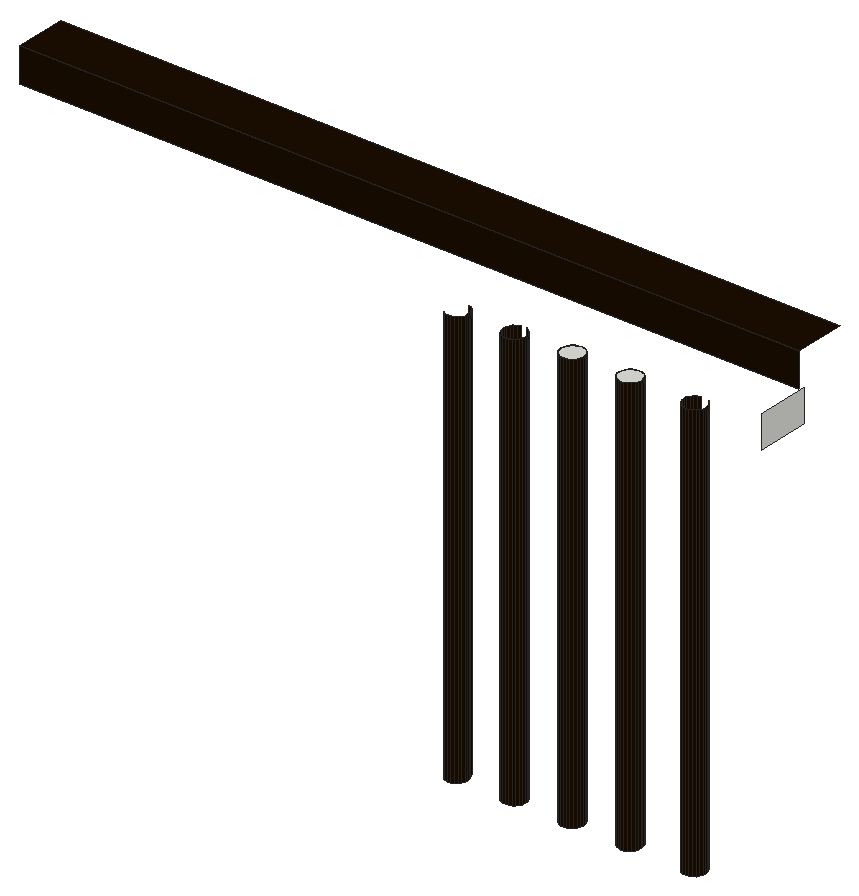
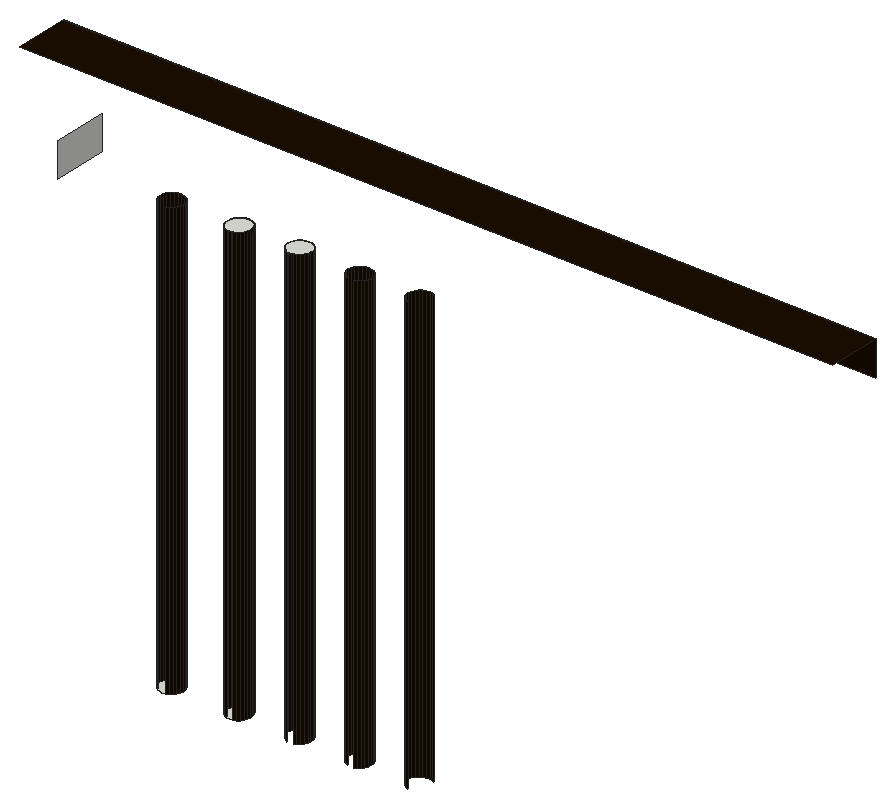
# SketchUp Ruby script. Lengths in inches.
U = 1.inch
M = Sketchup.active_model
def pt(a) = Geom::Point3d.new(a.map { |v| v * U })
def face(e, loops, mat)
  f = e.add_face(loops[0].map { |a| pt(a) })
  loops[1..].each { |l| e.add_face(l.map { |a| pt(a) }).erase! }
  f.material = f.back_material = mat if mat
  f
end
# faces: each face lists its corners as indices into pts; further lists are holes
def faces(e, pts, list, mat = nil) = list.each { |f| face(e, (f[0].is_a?(Array) ? f : [f]).map { |l| l.map { |i| pts[i] } }, mat) }
# xy, xz, yz: faces in a plane at the given z, y or x. An outline is a flat list of corners, or four numbers for a rectangle; further outlines are holes
def ring(l) = l.size == 4 ? [[l[0], l[1]], [l[2], l[1]], [l[2], l[3]], [l[0], l[3]]] : l.each_slice(2).to_a
def flat(e, list, mat, &to3) = list.each { |f| face(e, (f[0].is_a?(Array) ? f : [f]).map { |l| ring(l).map { |u, v| to3.(u, v) } }, mat) }
def xy(e, z, list, mat = nil) = flat(e, list, mat) { |x, y| [x, y, z] }
def xz(e, y, list, mat = nil) = flat(e, list, mat) { |x, z| [x, y, z] }
def yz(e, x, list, mat = nil) = flat(e, list, mat) { |y, z| [x, y, z] }
def lines(e, pts, list) = list.each { |a, b| e.add_line(pt(pts[a]), pt(pts[b])) }
# prism: a flat outline (further loops are holes) pulled along v
def prism(e, loops, v, mat = nil)
  f = face(e, loops, mat); d = Geom::Vector3d.new(v.map { |x| x * U })
  f.pushpull(f.normal.samedirection?(d) ? d.length : -d.length)
end
def box(e, o, s, mat = nil) = prism(e, [[o, [o[0] + s[0], o[1], o[2]], [o[0] + s[0], o[1] + s[1], o[2]], [o[0], o[1] + s[1], o[2]]]], [0, 0, s[2]], mat)
def at(x, y, z, deg = 0) = Geom::Transformation.translation(pt([x, y, z])) * Geom::Transformation.rotation(ORIGIN, Z_AXIS, deg.degrees)
def axes(o, x, y, z) = Geom::Transformation.new([*x, 0, *y, 0, *z, 0, *pt(o).to_a, 1])
def part(name) = M.definitions.add(name)
# library, detail: a bought-in or finely detailed component or shape, given as its bounding box
def library(name, o, s) = part(name).tap { |d| box(d.entities, o, s) }
def detail(e, o, s) = box(e.add_group.entities, o, s)
def put(e, d, t, mat = nil) = e.add_instance(d, t).tap { |i| i.material = mat if mat }
def group(e, t, mat = nil) = e.add_group.tap { |g| g.transformation = t; g.material = mat if mat }.entities
root = M.entities
M.materials.add("[Metal Seamed]1").color = [28, 14, 0]
xy(root,618.25,[[344.39,68.79,344.05,68.83,343.73,68.97,343.46,69.17,343.25,69.45,343.12,69.76,343.07,70.1,343.12,70.44,343.25,70.76,343.46,71.03,343.73,71.24,344.05,71.37,344.39,71.41,344.73,71.37,345.04,71.24,345.31,71.03,345.52,70.76,345.65,70.44,345.7,70.1,345.65,69.76,345.52,69.45,345.31,69.17,345.04,68.97,344.73,68.83],[351.89,68.79,351.55,68.83,351.23,68.97,350.96,69.17,350.75,69.45,350.62,69.76,350.58,70.1,350.62,70.44,350.75,70.76,350.96,71.03,351.23,71.24,351.55,71.37,351.89,71.41,352.23,71.37,352.55,71.24,352.82,71.03,353.03,70.76,353.16,70.44,353.2,70.1,353.16,69.76,353.03,69.45,352.82,69.17,352.55,68.97,352.23,68.83]])
xy(root,666.8125,[[344.39,68.79,344.73,68.83,345.04,68.97,345.31,69.17,345.52,69.45,345.65,69.76,345.7,70.1,345.65,70.44,345.52,70.76,345.31,71.03,345.04,71.24,344.73,71.37,344.39,71.41,344.05,71.37,343.73,71.24,343.46,71.03,343.25,70.76,343.12,70.44,343.07,70.1,343.12,69.76,343.25,69.45,343.46,69.17,343.73,68.97,344.05,68.83]])
xy(root,666.9375,[[337.7,68.79,338.04,68.83,338.36,68.97,338.63,69.17,338.84,69.45,338.97,69.76,339.01,70.1,338.97,70.44,338.84,70.76,338.63,71.03,338.36,71.24,338.04,71.37,337.7,71.41,337.36,71.37,337.04,71.24,336.77,71.03,336.5625,70.76,336.43,70.44,336.39,70.1,336.43,69.76,336.5625,69.45,336.77,69.17,337.04,68.97,337.36,68.83]])
xy(root,678.3125,[[275.92,67.28,366.15,73.28]],"[Metal Seamed]1")
xz(root,67.28,[[275.92,674.375,366.15,678.3125]],"[Metal Seamed]1")
yz(root,361.98,[[67.16,666.66,73.28,670.37]])
p = [[323.67,68.97,618.25],[323.98,68.83,618.25],[323.98,68.83,666.66],[323.67,68.97,666.66],[324.32,68.79,618.25],[324.32,68.79,666.66],
  [324.66,68.83,618.25],[324.66,68.83,666.66],[324.98,68.97,618.25],[324.98,68.97,666.66],[330.36,68.97,618.25],[330.67,68.83,618.25],
  [330.67,68.83,666.66],[330.36,68.97,666.66],[331.01,68.79,618.25],[331.01,68.79,666.66],[331.35,68.83,618.25],[331.35,68.83,666.66],
  [331.67,68.97,618.25],[331.67,68.97,666.66],[337.04,68.97,618.25],[337.36,68.83,618.25],[337.36,68.83,666.9375],[337.04,68.97,666.9375],
  [337.7,68.79,618.25],[337.7,68.79,666.9375],[338.04,68.83,618.25],[338.04,68.83,666.9375],[338.36,68.97,618.25],[338.36,68.97,666.9375],
  [343.73,68.97,618.25],[344.05,68.83,618.25],[344.05,68.83,666.8125],[343.73,68.97,666.8125],[344.39,68.79,618.25],[344.39,68.79,666.8125],
  [344.73,68.83,618.25],[344.73,68.83,666.8125],[345.04,68.97,618.25],[345.04,68.97,666.8125],[351.23,68.97,618.25],[351.55,68.83,618.25],
  [351.55,68.83,666.66],[351.23,68.97,666.66],[351.89,68.79,618.25],[351.89,68.79,666.66],[352.23,68.83,618.25],[352.23,68.83,666.66],
  [352.55,68.97,618.25],[352.55,68.97,666.66],[325.25,69.17,618.25],[325.25,69.17,666.66],[330.08,69.17,618.25],[330.08,69.17,666.66],
  [331.94,69.17,618.25],[331.94,69.17,666.66],[336.77,69.17,618.25],[336.77,69.17,666.9375],[338.63,69.17,618.25],[338.63,69.17,666.9375],
  [343.46,69.17,618.25],[343.46,69.17,666.8125],[345.31,69.17,618.25],[345.31,69.17,666.8125],[350.96,69.17,618.25],[350.96,69.17,666.66],
  [352.82,69.17,618.25],[352.82,69.17,666.66],[325.46,69.45,618.25],[325.46,69.45,666.66],[329.875,69.45,618.25],[329.875,69.45,666.66],
  [332.15,69.45,618.25],[332.15,69.45,666.66],[336.5625,69.45,618.25],[336.5625,69.45,666.9375],[338.84,69.45,618.25],[338.84,69.45,666.9375],
  [343.25,69.45,618.25],[343.25,69.45,666.8125],[345.52,69.45,618.25],[345.52,69.45,666.8125],[350.75,69.45,618.25],[350.75,69.45,666.66],
  [353.03,69.45,618.25],[353.03,69.45,666.66],[325.59,69.76,618.25],[325.59,69.76,666.66],[329.74,69.76,618.25],[329.74,69.76,666.66],
  [332.28,69.76,618.25],[332.28,69.76,666.66],[336.43,69.76,618.25],[336.43,69.76,666.9375],[338.97,69.76,618.25],[338.97,69.76,666.9375],
  [343.12,69.76,618.25],[343.12,69.76,666.8125],[345.65,69.76,618.25],[345.65,69.76,666.8125],[350.62,69.76,618.25],[350.62,69.76,666.66],
  [353.16,69.76,618.25],[353.16,69.76,666.66],[325.64,70.1,618.25],[325.64,70.1,666.66],[329.7,70.1,618.25],[329.7,70.1,666.66],
  [332.32,70.1,618.25],[332.32,70.1,666.66],[336.39,70.1,618.25],[336.39,70.1,666.9375],[339.01,70.1,618.25],[339.01,70.1,666.9375],
  [343.07,70.1,618.25],[343.07,70.1,666.8125],[345.7,70.1,618.25],[345.7,70.1,666.8125],[350.58,70.1,618.25],[350.58,70.1,666.66],
  [353.2,70.1,618.25],[353.2,70.1,666.66],[325.59,70.44,618.25],[325.59,70.44,666.66],[329.74,70.44,618.25],[329.74,70.44,666.66],
  [332.28,70.44,618.25],[332.28,70.44,666.66],[336.43,70.44,618.25],[336.43,70.44,666.9375],[338.97,70.44,618.25],[338.97,70.44,666.9375],
  [343.12,70.44,618.25],[343.12,70.44,666.8125],[345.65,70.44,618.25],[345.65,70.44,666.8125],[350.62,70.44,618.25],[350.62,70.44,666.66],
  [353.16,70.44,618.25],[353.16,70.44,666.66],[325.46,70.76,618.25],[325.46,70.76,666.66],[329.875,70.76,618.25],[329.875,70.76,666.66],
  [332.15,70.76,618.25],[332.15,70.76,666.66],[336.5625,70.76,618.25],[336.5625,70.76,666.9375],[338.84,70.76,618.25],[338.84,70.76,666.9375],
  [343.25,70.76,618.25],[343.25,70.76,666.8125],[345.52,70.76,618.25],[345.52,70.76,666.8125],[350.75,70.76,618.25],[350.75,70.76,666.66],
  [353.03,70.76,618.25],[353.03,70.76,666.66],[325.25,71.03,618.25],[325.25,71.03,666.66],[330.08,71.03,618.25],[330.08,71.03,666.66],
  [331.94,71.03,618.25],[331.94,71.03,666.66],[336.77,71.03,618.25],[336.77,71.03,666.9375],[338.63,71.03,618.25],[338.63,71.03,666.9375],
  [343.46,71.03,618.25],[343.46,71.03,666.8125],[345.31,71.03,618.25],[345.31,71.03,666.8125],[350.96,71.03,618.25],[350.96,71.03,666.66],
  [352.82,71.03,618.25],[352.82,71.03,666.66],[324.98,71.24,618.25],[324.98,71.24,666.66],[330.36,71.24,618.25],[330.36,71.24,666.66],
  [331.67,71.24,618.25],[331.67,71.24,666.66],[337.04,71.24,618.25],[337.04,71.24,666.9375],[338.36,71.24,618.25],[338.36,71.24,666.9375],
  [343.73,71.24,618.25],[343.73,71.24,666.8125],[345.04,71.24,618.25],[345.04,71.24,666.8125],[351.23,71.24,618.25],[351.23,71.24,666.66],
  [352.55,71.24,618.25],[352.55,71.24,666.66],[324.66,71.37,618.25],[324.66,71.37,666.66],[330.67,71.37,618.25],[330.67,71.37,666.66],
  [331.35,71.37,618.25],[331.35,71.37,666.66],[337.36,71.37,618.25],[337.36,71.37,666.9375],[338.04,71.37,618.25],[338.04,71.37,666.9375],
  [344.05,71.37,618.25],[344.05,71.37,666.8125],[344.73,71.37,618.25],[344.73,71.37,666.8125],[351.55,71.37,618.25],[351.55,71.37,666.66]]
faces(root,p,[[0,1,2,3],[1,4,5,2],[4,6,7,5],[6,8,9,7],[10,11,12,13],[11,14,15,12],[14,16,17,15],[16,18,19,17],
  [20,21,22,23],[21,24,25,22],[24,26,27,25],[26,28,29,27],[30,31,32,33],[31,34,35,32],[34,36,37,35],[36,38,39,37],
  [40,41,42,43],[41,44,45,42],[44,46,47,45],[46,48,49,47],[8,50,51,9],[52,10,13,53],[18,54,55,19],[56,20,23,57],
  [28,58,59,29],[60,30,33,61],[38,62,63,39],[64,40,43,65],[48,66,67,49],[50,68,69,51],[70,52,53,71],[54,72,73,55],
  [74,56,57,75],[58,76,77,59],[78,60,61,79],[62,80,81,63],[82,64,65,83],[66,84,85,67],[68,86,87,69],[88,70,71,89],
  [72,90,91,73],[92,74,75,93],[76,94,95,77],[96,78,79,97],[80,98,99,81],[100,82,83,101],[84,102,103,85],[86,104,105,87],
  [106,88,89,107],[90,108,109,91],[110,92,93,111],[94,112,113,95],[114,96,97,115],[98,116,117,99],[118,100,101,119],[102,120,121,103],
  [104,122,123,105],[124,106,107,125],[108,126,127,109],[128,110,111,129],[112,130,131,113],[132,114,115,133],[116,134,135,117],[136,118,119,137],
  [120,138,139,121],[122,140,141,123],[142,124,125,143],[126,144,145,127],[146,128,129,147],[130,148,149,131],[150,132,133,151],[134,152,153,135],
  [154,136,137,155],[138,156,157,139],[140,158,159,141],[160,142,143,161],[144,162,163,145],[164,146,147,165],[148,166,167,149],[168,150,151,169],
  [152,170,171,153],[172,154,155,173],[156,174,175,157],[158,176,177,159],[178,160,161,179],[162,180,181,163],[182,164,165,183],[166,184,185,167],
  [186,168,169,187],[170,188,189,171],[190,172,173,191],[174,192,193,175],[176,194,195,177],[196,178,179,197],[180,198,199,181],[200,182,183,201],
  [184,202,203,185],[204,186,187,205],[188,206,207,189],[208,190,191,209]],"[Metal Seamed]1")
